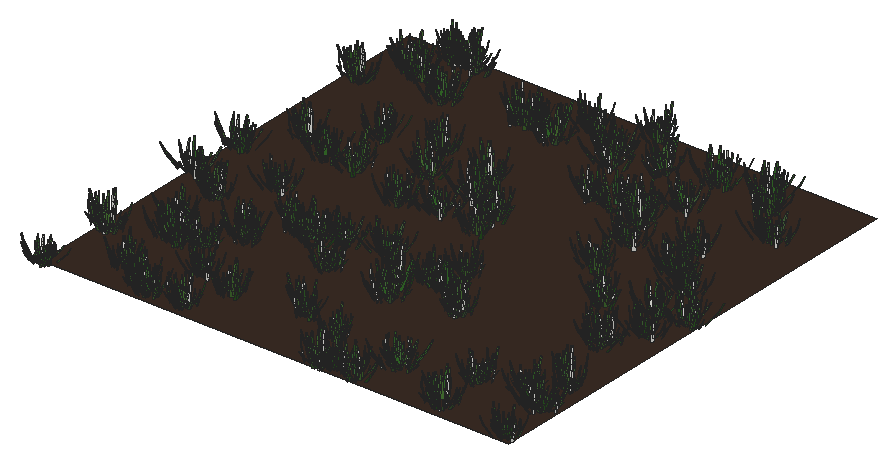
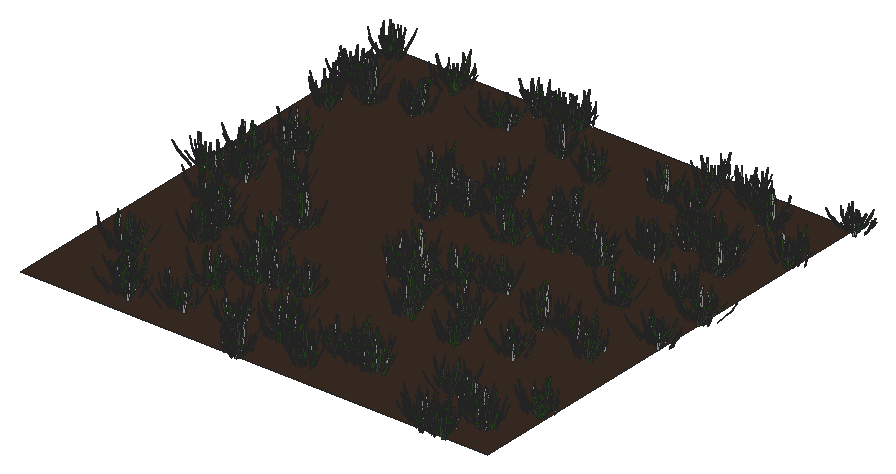
# SketchUp Ruby script. Lengths in inches.
U = 1.inch
M = Sketchup.active_model
def pt(a) = Geom::Point3d.new(a.map { |v| v * U })
def face(e, loops, mat)
  f = e.add_face(loops[0].map { |a| pt(a) })
  loops[1..].each { |l| e.add_face(l.map { |a| pt(a) }).erase! }
  f.material = f.back_material = mat if mat
  f
end
# faces: each face lists its corners as indices into pts; further lists are holes
def faces(e, pts, list, mat = nil) = list.each { |f| face(e, (f[0].is_a?(Array) ? f : [f]).map { |l| l.map { |i| pts[i] } }, mat) }
# xy, xz, yz: faces in a plane at the given z, y or x. An outline is a flat list of corners, or four numbers for a rectangle; further outlines are holes
def ring(l) = l.size == 4 ? [[l[0], l[1]], [l[2], l[1]], [l[2], l[3]], [l[0], l[3]]] : l.each_slice(2).to_a
def flat(e, list, mat, &to3) = list.each { |f| face(e, (f[0].is_a?(Array) ? f : [f]).map { |l| ring(l).map { |u, v| to3.(u, v) } }, mat) }
def xy(e, z, list, mat = nil) = flat(e, list, mat) { |x, y| [x, y, z] }
def xz(e, y, list, mat = nil) = flat(e, list, mat) { |x, z| [x, y, z] }
def yz(e, x, list, mat = nil) = flat(e, list, mat) { |y, z| [x, y, z] }
def lines(e, pts, list) = list.each { |a, b| e.add_line(pt(pts[a]), pt(pts[b])) }
# prism: a flat outline (further loops are holes) pulled along v
def prism(e, loops, v, mat = nil)
  f = face(e, loops, mat); d = Geom::Vector3d.new(v.map { |x| x * U })
  f.pushpull(f.normal.samedirection?(d) ? d.length : -d.length)
end
def box(e, o, s, mat = nil) = prism(e, [[o, [o[0] + s[0], o[1], o[2]], [o[0] + s[0], o[1] + s[1], o[2]], [o[0], o[1] + s[1], o[2]]]], [0, 0, s[2]], mat)
def at(x, y, z, deg = 0) = Geom::Transformation.translation(pt([x, y, z])) * Geom::Transformation.rotation(ORIGIN, Z_AXIS, deg.degrees)
def axes(o, x, y, z) = Geom::Transformation.new([*x, 0, *y, 0, *z, 0, *pt(o).to_a, 1])
def part(name) = M.definitions.add(name)
# library, detail: a bought-in or finely detailed component or shape, given as its bounding box
def library(name, o, s) = part(name).tap { |d| box(d.entities, o, s) }
def detail(e, o, s) = box(e.add_group.entities, o, s)
def put(e, d, t, mat = nil) = e.add_instance(d, t).tap { |i| i.material = mat if mat }
def group(e, t, mat = nil) = e.add_group.tap { |g| g.transformation = t; g.material = mat if mat }.entities
root = M.entities
M.materials.add("Material1").color = [58, 110, 58]
M.materials.add("Material10").color = [48, 100, 38]
M.materials.add("Material3").color = [68, 110, 58]
M.materials.add("Material4").color = [48, 90, 38]
M.materials.add("Material5").color = [68, 110, 48]
M.materials.add("Material6").color = [48, 90, 48]
M.materials.add("Material8").color = [58, 90, 38]
M.materials.add("Material9").color = [68, 100, 58]
M.materials.add("top-soil").color = [58, 44, 36]
c1 = part("grass00")
p = [[-0.6875,0.15,0],[-0.56,0.08,5.52],[-0.04,0.03,2.76],[0.48,-0.02,0],[0.35,-0.02,5.52],[-0.1,-0.14,5.52],
  [-0.12,0.65,8.37],[-0.42,0.65,8.37]]
faces(c1.entities,p,[[0,1,2,3],[3,2,4],[1,5,2],[5,4,2],[1,6,5],[4,5,6],[7,6,1]])
c2 = part("Group16\#1")
put(c2.entities,c1,axes([1.44,-0.61,-0.01],[0.05352,0.12609,0],[-0.10704,0.04543,0.07239],[0.06664,-0.02828,0.11628]),"Material6")
put(c2.entities,c1,axes([0.76,-0.15,-0.01],[0.04676,0.24062,0],[-0.23162,0.04501,0.06642],[0.0652,-0.01267,0.23595]),"Material3")
put(c2.entities,c1,axes([0.79,0.01,-0.01],[-0.00606,0.34651,0],[-0.34381,-0.00602,0.0432],[0.04319,0.00076,0.34386]))
put(c2.entities,c1,axes([1,0.23,-0.01],[-0.07192,0.31144,0],[-0.28722,-0.06632,0.1236],[0.12043,0.02781,0.29478]),"Material5")
put(c2.entities,c1,axes([1.66,0.77,-0.01],[-0.13828,0.29651,0],[-0.21551,-0.1005,0.22471],[0.20365,0.09498,0.23779]),"Material10")
put(c2.entities,c1,axes([0.6875,0.52,-0.01],[-0.18126,0.24051,0],[-0.22746,-0.17142,0.09788],[0.07817,0.05891,0.28481]),"Material5")
put(c2.entities,c1,axes([0.68,0.78,-0.01],[-0.215,0.18688,0],[-0.12385,-0.14248,0.21334],[0.13995,0.16101,0.18878]),"Material3")
put(c2.entities,c1,axes([0.56,1,-0.01],[-0.13756,0.07624,0],[-0.06159,-0.11112,0.0927],[0.04494,0.08108,0.12705]),"Material5")
put(c2.entities,c1,axes([0.2,0.64,-0.01],[-0.23729,0.07254,0],[-0.05711,-0.18681,0.153],[0.04473,0.14632,0.19535]),"Material10")
put(c2.entities,c1,axes([0.0625,0.72,-0.01],[-0.28874,0.02525,0],[-0.02179,-0.24916,0.14647],[0.01276,0.14591,0.25012]),"Material3")
put(c2.entities,c1,axes([-0.08,0.62,-0.01],[-0.34089,-0.04187,0],[0.03255,-0.26504,0.216],[-0.02633,0.21439,0.26703]),"Material10")
put(c2.entities,c1,axes([-0.34,0.98,-0.01],[-0.14314,-0.0493,0],[0.04397,-0.12769,0.06843],[-0.02228,0.0647,0.13505]),"Material10")
put(c2.entities,c1,axes([-0.87,1.45,-0.01],[-0.23488,-0.14114,0],[0.13761,-0.22901,0.06087],[-0.03135,0.05217,0.26717]))
put(c2.entities,c1,axes([-0.72,0.77,-0.01],[-0.14208,-0.13251,0],[0.07209,-0.0773,0.16301],[-0.11118,0.11922,0.1057]),"Material10")
put(c2.entities,c1,axes([-0.62,0.43,-0.01],[-0.14845,-0.21203,0],[0.18654,-0.13061,0.12304],[-0.10079,0.07057,0.22772]),"Material3")
put(c2.entities,c1,axes([-0.68,0.29,-0.01],[-0.13639,-0.32136,0],[0.31723,-0.13464,0.05579],[-0.05136,0.0218,0.34462]),"Material4")
put(c2.entities,c1,axes([-0.64,0.125,-0.01],[-0.0458,-0.23569,0],[0.22124,-0.043,0.08276],[-0.08124,0.01579,0.22538]),"Material1")
put(c2.entities,c1,axes([-1.6,-0.03,-0.01],[0.00576,-0.32897,0],[0.27526,0.00482,0.18018],[-0.18015,-0.00315,0.2753]),"Material5")
put(c2.entities,c1,axes([-1.36,-0.31,-0.01],[0.05718,-0.24765,0],[0.18172,0.04196,0.17267],[-0.16825,-0.03885,0.1865]),"Material10")
put(c2.entities,c1,axes([-1.54,-0.72,-0.01],[0.06537,-0.14017,0],[0.13555,0.06321,0.03939],[-0.0357,-0.01665,0.14956]))
put(c2.entities,c1,axes([-1.19,-0.9,-0.01],[0.09597,-0.12735,0],[0.11214,0.08451,0.07557],[-0.06035,-0.04548,0.14042]),"Material9")
put(c2.entities,c1,axes([-0.47,-0.54,-0.01],[0.11588,-0.10072,0],[0.0618,0.0711,0.12124],[-0.07953,-0.0915,0.0942]))
put(c2.entities,c1,axes([-0.47,-0.84,-0.01],[0.11927,-0.0661,0],[0.06603,0.11913,0.00646],[-0.00313,-0.00565,0.13621]),"Material5")
put(c2.entities,c1,axes([-0.38,-1.24,-0.01],[0.28037,-0.08571,0],[0.0618,0.20215,0.20315],[-0.05939,-0.19428,0.21139]),"Material9")
put(c2.entities,c1,axes([-0.06,-0.66,-0.01],[0.22719,-0.01987,0],[0.01247,0.14255,0.17758],[-0.01547,-0.17691,0.1431]),"Material8")
put(c2.entities,c1,axes([0.11,-0.89,-0.01],[0.14882,0.01828,0],[-0.01058,0.08611,0.12229],[0.01491,-0.12138,0.08676]),"Material6")
put(c2.entities,c1,axes([0.25,-0.72,-0.01],[0.20481,0.07053,0],[-0.06206,0.18022,0.10291],[0.03351,-0.0973,0.1906]),"Material6")
put(c2.entities,c1,axes([0.85,-1.42,-0.01],[0.16481,0.09904,0],[-0.09472,0.15762,0.05616],[0.02893,-0.04814,0.18389]),"Material5")
put(c2.entities,c1,axes([1.01,-1.09,-0.01],[0.21858,0.20385,0],[-0.17495,0.1876,0.15339],[0.10462,-0.11218,0.25652]),"Material10")
put(c2.entities,c1,axes([1.01,-0.71,-0.01],[0.08733,0.12473,0],[-0.06445,0.04512,0.13037],[0.1068,-0.07477,0.07867]),"Material6")
c3 = part("Group15\#1")
put(c3.entities,c2,at(0,0,0))
c4 = part("3darcstudiotree_grass00\#1")
put(c4.entities,c3,at(0,0,0))
xy(root,0.25,[[266.29,97.01,332.83,162.37]],"top-soil")
put(root,c4,axes([309.93,98.23,0.25],[0.86121,-0.44279,0],[0.5071,0.67945,-0.00486],[0.00379,0.00508,1.42853]))
put(root,c4,axes([312.83,145.03,0.25],[-0.52266,0.74393,0],[-1.03411,-0.50051,-0.00159],[-0.00186,-0.0009,1.61385]))
put(root,c4,axes([329.97,111.25,0.25],[-0.2859,0.83391,0],[-0.89169,-0.2106,-0.00052],[-0.00091,-0.00021,1.67384]))
put(root,c4,axes([283.98,120.42,0.25],[-0.76285,0.6241,0],[-0.83432,-0.70254,-0.00446],[-0.00381,-0.00321,1.44777]))
put(root,c4,axes([284.78,99.1875,0.25],[0.12915,0.86215,0],[-0.96561,0.09965,-0.00588],[-0.00819,0.00085,1.36568]))
put(root,c4,axes([323.6875,138.39,0.25],[-0.98277,-0.04412,0],[0.05146,-0.78971,-0.00522],[0.00041,-0.00637,1.40302]))
put(root,c4,axes([271.18,156.96,0.25],[0.29935,-0.91019,0],[1.13241,0.25657,-0.00598],[0.00666,0.00151,1.35627]))
put(root,c4,axes([290.08,154.99,0.25],[0.93627,0.12764,0],[-0.15967,0.80684,-0.00501],[-0.00116,0.00588,1.40942]))
put(root,c4,axes([302.36,153.3,0.25],[-1.12691,0.04818,0],[-0.05925,-0.95478,-0.00589],[-0.00036,-0.00576,1.35922]))
put(root,c4,axes([285.51,144.52,0.25],[-0.12809,0.73941,0],[-1.04403,-0.12459,-0.00494],[-0.00655,-0.00078,1.4129]))
put(root,c4,axes([271.8125,137.39,0.25],[-0.38292,0.95693,0],[-1.03559,-0.28548,-0.00679],[-0.00772,-0.00213,1.30662]))
put(root,c4,axes([267.22,123.47,0.25],[-1.29158,0.07845,0],[-0.08531,-0.96753,-0.0067],[-0.00055,-0.00621,1.30916]))
put(root,c4,axes([287.36,139.38,0.25],[0.94797,-0.50383,0],[0.61806,0.80111,-0.00312],[0.00222,0.00288,1.51309]))
put(root,c4,axes([305.24,146.21,0.25],[-0.87234,0.36685,0],[-0.4401,-0.72094,-0.00642],[-0.00394,-0.00646,1.3229]))
put(root,c4,axes([315.26,134.25,0.25],[-0.10317,-0.82288,0],[1.26583,-0.10933,-0.00351],[0.00407,-0.00035,1.48465]))
put(root,c4,axes([274.2,101.96,0.25],[0.39841,-0.78569,0],[0.91997,0.32138,-0.00467],[0.00612,0.00214,1.41828]))
put(root,c4,axes([322.18,139.6875,0.25],[-0.34498,-0.76417,0],[1.21423,-0.37762,-0.00645],[0.00613,-0.00191,1.31612]))
put(root,c4,axes([288.96,132.18,0.25],[0.79894,0.62733,0],[-0.77291,0.67811,-0.00432],[-0.00378,0.00332,1.43292]))
put(root,c4,axes([331.41,98.26,0.25],[-0.80376,-0.40476,0],[0.5718,-0.78221,-0.00574],[0.00364,-0.00497,1.3472]))
put(root,c4,axes([326.9375,130.1,0.25],[0.99644,0.23212,0],[-0.24487,0.72413,-0.00495],[-0.00205,0.00607,1.38942]))
put(root,c4,axes([267.36,107.35,0.25],[0.18541,0.80242,0],[-1.21307,0.1931,-0.00068],[-0.00088,0.00014,1.62852]))
put(root,c4,axes([295.38,158.58,0.25],[-0.7805,-0.38541,0],[0.66159,-0.92299,-0.00321],[0.00188,-0.00262,1.48019]))
put(root,c4,axes([299.28,155.89,0.25],[-0.92169,0.64984,0],[-0.59274,-0.57917,-0.00331],[-0.00346,-0.00338,1.47415]))
put(root,c4,axes([320.93,128.45,0.25],[0.6856,-0.64948,0],[0.72334,0.52602,-0.00209],[0.00252,0.00183,1.54397]))
put(root,c4,axes([280.28,135.0625,0.25],[0.18578,-1.05764,0],[1.2528,0.1516,-0.00277],[0.00324,0.00039,1.49508]))
put(root,c4,axes([305.1,97.96,0.25],[-0.03906,0.78462,0],[-1.12299,-0.03851,-0.00296],[-0.0039,-0.00013,1.47961]))
put(root,c4,axes([307.5625,156.03,0.25],[0.18691,1.0512,0],[-0.89716,0.10989,-0.00575],[-0.00828,0.00101,1.31904]))
put(root,c4,axes([275.26,109.78,0.25],[1.19617,-0.31577,0],[0.29503,0.76992,-0.00335],[0.00152,0.00396,1.45436]))
put(root,c4,axes([282.34,105.79,0.25],[-0.8751,-0.26339,0],[0.33277,-0.76166,-0.00444],[0.00216,-0.00494,1.39182]))
put(root,c4,axes([287.4,104.39,0.25],[0.36018,-0.73027,0],[1.01794,0.34587,-0.00546],[0.00612,0.00208,1.33158]))
put(root,c4,axes([273.36,155.75,0.25],[0.50995,-0.74136,0],[0.96885,0.4591,-0.00497],[0.00525,0.00249,1.35772]))
put(root,c4,axes([295.19,138.06,0.25],[-1.19058,0.17726,0],[-0.21867,-1.01181,-0.00093],[-0.00021,-0.00097,1.58752]))
put(root,c4,axes([301.6,114.58,0.25],[0.55171,0.95492,0],[-0.97206,0.38689,-0.00104],[-0.00137,0.00054,1.58037]))
put(root,c4,axes([326.93,151.08,0.25],[-1.1964,-0.25343,0],[0.22268,-0.72421,-0.00096],[0.00042,-0.00135,1.58162]))
put(root,c4,axes([288.54,154.77,0.25],[-0.75443,0.67184,0],[-0.85399,-0.66064,-0.00031],[-0.00032,-0.00025,1.61707]))
put(root,c4,axes([293.47,153.96,0.25],[0.45478,0.93849,0],[-1.06156,0.35438,-0.0015],[-0.00188,0.00063,1.54039]))
put(root,c4,axes([301.16,155.96,0.25],[-1.00861,-0.01357,0],[0.01665,-0.85218,-0.00434],[0.00009,-0.00483,1.37632]))
put(root,c4,axes([285.41,119.9,0.25],[0.10289,-0.76682,0],[1.10968,0.10257,-0.00391],[0.00486,0.00045,1.39627]))
put(root,c4,axes([273.47,161.36,0.25],[-0.326,0.90661,0],[-0.89785,-0.22242,-0.00408],[-0.00578,-0.00143,1.38631]))
put(root,c4,axes([278.05,111.15,0.25],[-0.44851,-0.78419,0],[0.95628,-0.37678,-0.00409],[0.00483,-0.0019,1.3842]))
put(root,c4,axes([275.3,161.52,0.25],[0.33745,0.78827,0],[-0.92185,0.27186,-0.0026],[-0.00367,0.00108,1.46428]))
put(root,c4,axes([329.91,105.42,0.25],[-1.03269,0.02174,0],[-0.02843,-0.93035,-0.00196],[-0.00007,-0.00217,1.49745]))
put(root,c4,axes([314.23,157.46,0.25],[1.14807,0.374,0],[-0.39385,0.83289,-0.00074],[-0.00039,0.00083,1.56313]))
put(root,c4,axes([321.15,106.22,0.25],[-0.21202,-0.91699,0],[0.93697,-0.14924,-0.00431],[0.00598,-0.00095,1.34772]))
put(root,c4,axes([305.28,123.74,0.25],[0.02691,-0.80536,0],[0.97679,0.02249,-0.00183],[0.00277,0.00006,1.48199]))
put(root,c4,axes([326.66,122.04,0.25],[0.2786,0.79282,0],[-1.16767,0.28267,-0.00405],[-0.00433,0.00105,1.35389]))
put(root,c4,axes([293.55,142.5,0.25],[-0.50455,0.88883,0],[-1.01115,-0.39542,-0.00165],[-0.00199,-0.00078,1.48801]))
put(root,c4,axes([267.3,130.81,0.25],[1.15659,0.00324,0],[-0.00316,0.77597,-0.00416],[-0.00002,0.00494,1.3392]))
put(root,c4,axes([306.64,98.52,0.25],[-0.70281,-0.50491,0],[0.75525,-0.72422,-0.00422],[0.00319,-0.00306,1.33295]))
put(root,c4,axes([292.14,115.66,0.25],[-0.36631,-0.75419,0],[0.98709,-0.33028,-0.00075],[0.00099,-0.00033,1.52674]))
put(root,c4,axes([326.41,120.62,0.25],[0.97536,-0.54489,0],[0.51207,0.63145,-0.0013],[0.00118,0.00146,1.49257]))
put(root,c4,axes([302.61,161.3125,0.25],[0.08585,-0.97173,0],[0.94331,0.05741,-0.00239],[0.0036,0.00022,1.42634]))
put(root,c4,axes([312.23,102.98,0.25],[1.04618,0.63702,0],[-0.65143,0.73702,-0.00415],[-0.00295,0.00334,1.32509]))
put(root,c4,axes([272.34,113.69,0.25],[0.40805,-0.74659,0],[1.10018,0.41424,-0.00454],[0.00445,0.00168,1.30224]))
put(root,c4,axes([331.17,130.67,0.25],[1.26584,0.24012,0],[-0.22903,0.83176,-0.00333],[-0.00099,0.00359,1.36941]))
put(root,c4,axes([278.33,153.3,0.25],[0.91305,0.67717,0],[-0.73512,0.68283,-0.00121],[-0.00109,0.00101,1.48985]))
put(root,c4,axes([280.14,98.55,0.25],[0.771,0.39895,0],[-0.49755,0.66242,-0.0044],[-0.00324,0.00431,1.30779]))
put(root,c4,axes([281.08,114.91,0.25],[0.76055,0.41822,0],[-0.69431,0.86982,-0.00365],[-0.00216,0.00271,1.34685]))
put(root,c4,axes([326.92,107.4,0.25],[0.05723,-0.98397,0],[1.06645,0.04273,-0.00402],[0.00499,0.0002,1.3243]))
put(root,c4,axes([278.39,99.62,0.25],[-0.19819,0.98714,0],[-0.89796,-0.1242,-0.00349],[-0.00512,-0.00071,1.35435]))
put(root,c4,axes([290.15,120.98,0.25],[-1.1706,-0.00557,0],[0.0054,-0.78085,-0.00073],[0.00001,-0.00097,1.50826]))
put(root,c4,axes([308.58,146.47,0.25],[1.03264,-0.42726,0],[0.56018,0.9327,-0.00236],[0.00118,0.00196,1.40454]))
put(root,c4,axes([329.42,125.79,0.25],[-1.09534,-0.33411,0],[0.35001,-0.7905,-0.00277],[0.0013,-0.00293,1.38049]))
put(root,c4,axes([321.73,143.79,0.25],[-0.82009,-0.58498,0],[0.66888,-0.64598,-0.00129],[0.0012,-0.00116,1.46122]))
put(root,c4,axes([276.43,134.85,0.25],[0.89718,0.41884,0],[-0.54336,0.80181,-0.00275],[-0.00167,0.00247,1.37565]))
put(root,c4,axes([314.96,140.67,0.25],[-1.09635,-0.30423,0],[0.28969,-0.71918,-0.00172],[0.00085,-0.00211,1.42531]))
put(root,c4,axes([309.86,116.75,0.25],[0.16665,0.828,0],[-0.92592,0.12838,-0.00028],[-0.00045,0.00006,1.50491]))
put(root,c4,axes([321.3,99.51,0.25],[-0.04627,1.02449,0],[-1.18428,-0.03685,-0.00219],[-0.00258,-0.00008,1.39308]))
put(root,c4,axes([311.45,147.7,0.25],[-0.87449,0.48266,0],[-0.57426,-0.71677,-0.00165],[-0.00125,-0.00156,1.42237]))
put(root,c4,axes([279.98,115.52,0.25],[0.91504,0.07643,0],[-0.11795,0.97282,-0.00091],[-0.00011,0.00093,1.45853]))
put(root,c4,axes([296.66,105.99,0.25],[-0.91339,0.74263,0],[-0.64153,-0.54357,-0.00183],[-0.00196,-0.00166,1.40539]))
put(root,c4,axes([305.99,119.51,0.25],[-1.23628,0.1981,0],[-0.20569,-0.88433,-0.00152],[-0.00038,-0.00161,1.41339]))
put(root,c4,axes([276.73,126.1875,0.25],[-0.98464,-0.25712,0],[0.34271,-0.90413,-0.00258],[0.00092,-0.00242,1.35273]))
put(root,c4,axes([287.31,119.29,0.25],[0.90353,-0.39739,0],[0.56525,0.88538,-0.00115],[0.00063,0.00099,1.42878]))
put(root,c4,axes([314.77,150.87,0.25],[-1.0977,-0.17705,0],[0.23835,-1.01804,-0.00093],[0.0002,-0.00087,1.42207]))
put(root,c4,axes([299.83,132.65,0.25],[0.45744,-0.92326,0],[1.03567,0.3535,-0.00107],[0.00124,0.00042,1.41133]))
put(root,c4,axes([299.41,136.41,0.25],[0.6975,-0.75634,0],[0.82019,0.52107,-0.00025],[0.00028,0.00018,1.45509]))
put(root,c4,axes([327,136.08,0.25],[-1.0933,-0.28437,0],[0.29294,-0.77586,-0.00157],[0.00066,-0.00175,1.37913]))
put(root,c4,axes([267.91,151.28,0.25],[-0.06108,0.74714,0],[-1.20058,-0.06761,-0.00038],[-0.00046,-0.00003,1.44006]))
put(root,c4,axes([276.99,160.88,0.25],[-1.12042,0.35052,0],[-0.36113,-0.79523,-0.00238],[-0.00108,-0.00238,1.31717]))
put(root,c4,axes([273.59,110.35,0.25],[0.90214,0.40636,0],[-0.61502,0.9406,-0.00178],[-0.00089,0.00135,1.34491]))
put(root,c4,axes([322.27,156.37,0.25],[-0.53873,0.622,0],[-0.90288,-0.53872,-0.0015],[-0.00148,-0.00088,1.35234]))
put(root,c4,axes([320.52,158.79,0.25],[1.1456,0.15924,0],[-0.19958,0.98911,-0.00046],[-0.00009,0.00044,1.40239]))
put(root,c4,axes([302.72,120.46,0.25],[0.40285,-0.76408,0],[0.82658,0.30023,-0.00213],[0.00282,0.00102,1.30651]))
put(root,c4,axes([270.98,156.53,0.25],[0.91392,-0.58858,0],[0.55525,0.59394,-0.00126],[0.00114,0.00122,1.3431]))
put(root,c4,axes([293.98,133.11,0.25],[-1.26073,-0.10303,0],[0.11515,-0.97068,-0.00134],[0.00015,-0.00126,1.33719]))
put(root,c4,axes([330.88,105.5,0.25],[-0.64625,-0.86587,0],[0.7697,-0.39575,-0.00146],[0.00182,-0.00093,1.32424]))
put(root,c4,axes([278.26,142.59,0.25],[0.93244,0.06191,0],[-0.09546,0.9904,-0.00093],[-0.00008,0.00087,1.35201]))
put(root,c4,axes([299.93,118.53,0.25],[-0.23154,0.76987,0],[-0.98482,-0.20404,-0.00012],[-0.00015,-0.00003,1.39497]))
put(root,c4,axes([272.07,120.66,0.25],[0.29464,0.74671,0],[-1.01807,0.27674,-0.00037],[-0.00045,0.00012,1.37352]))
put(root,c4,axes([295.21,122.6,0.25],[-1.11889,-0.35173,0],[0.44595,-0.97728,-0.00084],[0.00032,-0.00069,1.34285]))
put(root,c4,axes([302.87,103.58,0.25],[0.34641,-0.83075,0],[0.8557,0.24581,-0.00044],[0.00061,0.00018,1.32507]))
put(root,c4,axes([266.29,97.01,0.25],[1,0,0],[0,0.83,0],[0,0,1]))
